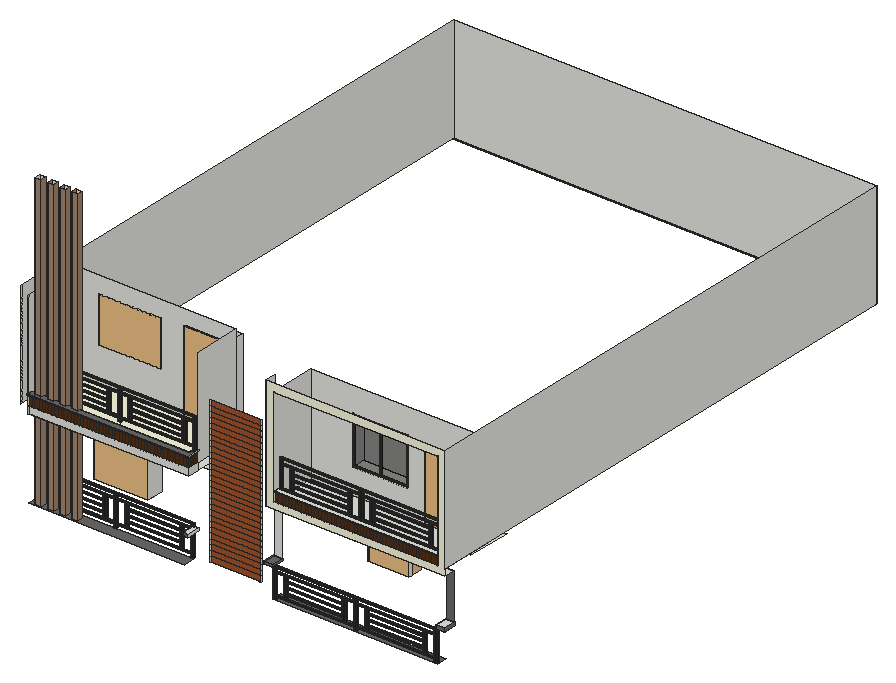
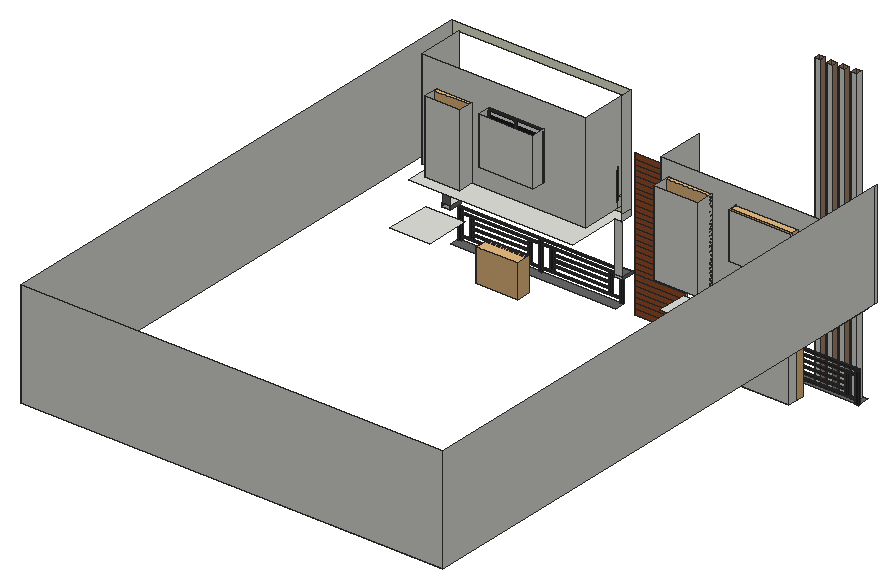
# SketchUp Ruby script. Lengths in inches.
U = 1.inch
M = Sketchup.active_model
def pt(a) = Geom::Point3d.new(a.map { |v| v * U })
def face(e, loops, mat)
  f = e.add_face(loops[0].map { |a| pt(a) })
  loops[1..].each { |l| e.add_face(l.map { |a| pt(a) }).erase! }
  f.material = f.back_material = mat if mat
  f
end
# faces: each face lists its corners as indices into pts; further lists are holes
def faces(e, pts, list, mat = nil) = list.each { |f| face(e, (f[0].is_a?(Array) ? f : [f]).map { |l| l.map { |i| pts[i] } }, mat) }
# xy, xz, yz: faces in a plane at the given z, y or x. An outline is a flat list of corners, or four numbers for a rectangle; further outlines are holes
def ring(l) = l.size == 4 ? [[l[0], l[1]], [l[2], l[1]], [l[2], l[3]], [l[0], l[3]]] : l.each_slice(2).to_a
def flat(e, list, mat, &to3) = list.each { |f| face(e, (f[0].is_a?(Array) ? f : [f]).map { |l| ring(l).map { |u, v| to3.(u, v) } }, mat) }
def xy(e, z, list, mat = nil) = flat(e, list, mat) { |x, y| [x, y, z] }
def xz(e, y, list, mat = nil) = flat(e, list, mat) { |x, z| [x, y, z] }
def yz(e, x, list, mat = nil) = flat(e, list, mat) { |y, z| [x, y, z] }
def lines(e, pts, list) = list.each { |a, b| e.add_line(pt(pts[a]), pt(pts[b])) }
# prism: a flat outline (further loops are holes) pulled along v
def prism(e, loops, v, mat = nil)
  f = face(e, loops, mat); d = Geom::Vector3d.new(v.map { |x| x * U })
  f.pushpull(f.normal.samedirection?(d) ? d.length : -d.length)
end
def box(e, o, s, mat = nil) = prism(e, [[o, [o[0] + s[0], o[1], o[2]], [o[0] + s[0], o[1] + s[1], o[2]], [o[0], o[1] + s[1], o[2]]]], [0, 0, s[2]], mat)
def at(x, y, z, deg = 0) = Geom::Transformation.translation(pt([x, y, z])) * Geom::Transformation.rotation(ORIGIN, Z_AXIS, deg.degrees)
def axes(o, x, y, z) = Geom::Transformation.new([*x, 0, *y, 0, *z, 0, *pt(o).to_a, 1])
def part(name) = M.definitions.add(name)
# library, detail: a bought-in or finely detailed component or shape, given as its bounding box
def library(name, o, s) = part(name).tap { |d| box(d.entities, o, s) }
def detail(e, o, s) = box(e.add_group.entities, o, s)
def put(e, d, t, mat = nil) = e.add_instance(d, t).tap { |i| i.material = mat if mat }
def group(e, t, mat = nil) = e.add_group.tap { |g| g.transformation = t; g.material = mat if mat }.entities
root = M.entities
M.materials.add("Glass_Tinted_Gray").color = [0, 0, 0]
M.materials["Glass_Tinted_Gray"].alpha = 0.125
M.materials.add("Painted Metal Railing").color = [35, 35, 35]
M.materials.add("Teddy_BraceletShadow ").color = [165, 134, 109]
M.materials.add("[0042_Sienna]").color = [160, 82, 45]
M.materials.add("[0049_Beige]").color = [245, 245, 220]
M.materials.add("[0134_DimGray]").color = [105, 105, 105]
M.materials.add("[0135_DarkGray]").color = [81, 81, 81]
M.materials.add("[Mirror 02]").color = [229, 229, 229]
M.materials.add("[Terrazzo Light Blue]").color = [196, 214, 227]
M.materials.add("[Wood Cherry Original]").color = [86, 49, 23]
c1 = part("Post")
box(c1.entities,[-0.75,-0.75,0],[1.5,1.5,34.5],"Painted Metal Railing")
c2 = part("Group43\#1")
box(c2.entities,[-0.75,0,0],[1.5,73.5,1.5],"Painted Metal Railing")
c3 = part("Group46\#2")
box(c3.entities,[-0.75,0.75,0],[1.5,34.5,1.5],"Painted Metal Railing")
c4 = part("Group49\#1")
box(c4.entities,[-0.75,0.75,0],[1.5,34.5,1.5],"Painted Metal Railing")
c5 = part("Group52\#1")
box(c5.entities,[-0.75,0.75,0],[1.5,34.5,1.5],"Painted Metal Railing")
c6 = part("Group55\#1")
box(c6.entities,[-0.75,0.75,0],[1.5,34.5,1.5],"Painted Metal Railing")
c7 = part("Inner Post")
box(c7.entities,[-0.75,-0.75,0],[1.5,1.5,23.5],"Painted Metal Railing")
c8 = part("Group59\#1")
box(c8.entities,[-0.75,0.75,0],[1.5,24.5,1.5],"Painted Metal Railing")
c9 = part("Group62\#1")
box(c9.entities,[-0.75,0.75,0],[1.5,24.5,1.5],"Painted Metal Railing")
c10 = part("Group65\#1")
box(c10.entities,[-0.75,0.75,0],[1.5,24.5,1.5],"Painted Metal Railing")
c11 = part("Inner Posts and Rails\#2")
put(c11.entities,c7,at(0,0,0,90))
put(c11.entities,c7,at(0,26,0,90))
put(c11.entities,c8,at(0,0,4.75))
put(c11.entities,c9,at(0,0,11))
put(c11.entities,c10,at(0,0,17.25))
c12 = part("Group69\#1")
box(c12.entities,[-0.75,0.75,0],[1.5,24.5,1.5],"Painted Metal Railing")
c13 = part("Group72\#1")
box(c13.entities,[-0.75,0.75,0],[1.5,24.5,1.5],"Painted Metal Railing")
c14 = part("Group75\#1")
box(c14.entities,[-0.75,0.75,0],[1.5,24.5,1.5],"Painted Metal Railing")
c15 = part("Inner Posts and Rails\#3")
put(c15.entities,c7,at(0,0,0,90))
put(c15.entities,c7,at(0,26,0,90))
put(c15.entities,c12,at(0,0,4.75))
put(c15.entities,c13,at(0,0,11))
put(c15.entities,c14,at(0,0,17.25))
c16 = part("Railing Assembly 14\#1")
put(c16.entities,c1,at(0,0,0))
put(c16.entities,c1,at(36,0,0))
put(c16.entities,c1,at(72,0,0))
put(c16.entities,c2,at(-0.75,0,34.5,-90))
put(c16.entities,c3,at(0,0,4,-90))
put(c16.entities,c4,at(36,0,4,-90))
put(c16.entities,c5,at(0,0,29,-90))
put(c16.entities,c6,at(36,0,29,-90))
put(c16.entities,c11,at(5,0,5.5,-90))
put(c16.entities,c15,at(41,0,5.5,-90))
c17 = library("Group\#6",[0,0,0],[8.07,62.0625,54])
c18 = library("PINTU 6 YA",[0,-0.6875,0],[35.83,8.07,80.71])
c19 = part("PENTEK_RP Fineline 50S_Sliding_DoorCase_E1")
box(c19.entities,[0,0,0],[1.51,3.66,99.27],"[0135_DarkGray]")
c20 = part("PENTEK_RP Fineline 50S_SlidingDooe_Case_E2")
box(c20.entities,[0,0,0],[96.25,3.66,1.51],"[0135_DarkGray]")
c21 = part("pentek_RP Fineline 50S_SlidingDoor_Case")
put(c21.entities,c19,at(97.76,0,0))
put(c21.entities,c20,at(1.51,0,0))
put(c21.entities,c19,at(0,0,0))
put(c21.entities,c20,at(1.51,0,97.76))
c22 = part("PENTEK_RP Fineline 50S_SlidingDoor_GlazingBead_2")
box(c22.entities,[0,0,0],[0.56,0.59,94.39],"[0135_DarkGray]")
c23 = part("PENTEK_RP Fineline 50S_SlidingDoor_Glass")
box(c23.entities,[0,0,0],[46.58,0.16,94.39],"Glass_Tinted_Gray")
c24 = part("PENTEK_RP Fineline 50S_SlidingDoor_GlazingBead")
box(c24.entities,[0,0,0],[45.47,0.59,0.56],"[0135_DarkGray]")
c25 = part("PENTEK_RP Fineline 50S_SlidingDoor_Leaf_E1")
xy(c25.entities,0,[[0,0,0.93,1.97],[0.93,1.57,1.49,1.97]],"[0135_DarkGray]")
xy(c25.entities,96.25,[[0,0,0.93,0,0.93,1.57,1.49,1.57,1.49,1.97,0,1.97]],"[0135_DarkGray]")
xz(c25.entities,0,[[0,0,0.93,96.25]],"[0135_DarkGray]")
xz(c25.entities,1.57,[[0.93,0,1.49,95.32],[0.93,95.32,1.49,96.25]],"[0135_DarkGray]")
xz(c25.entities,1.97,[[0,0,1.49,96.25]],"[0135_DarkGray]")
yz(c25.entities,0,[[0,0,1.97,96.25]],"[0135_DarkGray]")
yz(c25.entities,0.93,[[0,0,1.57,0.93],[0,0.93,1.57,95.32],[0,95.32,1.57,96.25]],"[0135_DarkGray]")
yz(c25.entities,1.49,[[1.57,0,1.97,95.32],[1.57,95.32,1.97,96.25]],"[0135_DarkGray]")
c26 = part("PENTEK_RP Fineline 50S_SlidingDoor_Leaf_E2")
xy(c26.entities,0,[[0,0,0,1.57,0.56,1.57,0.56,1.97,46.02,1.97,46.02,1.57,46.58,1.57,46.58,0]],"[0135_DarkGray]")
xy(c26.entities,0.93,[[0,0,46.58,1.57]],"[0135_DarkGray]")
xy(c26.entities,1.49,[[0.56,1.57,46.02,1.97]],"[0135_DarkGray]")
xz(c26.entities,0,[[0,0,46.58,0.93]],"[0135_DarkGray]")
xz(c26.entities,1.57,[[0,0,0.56,0.93],[46.02,0,46.58,0.93],[0.56,0.93,46.02,1.49]],"[0135_DarkGray]")
xz(c26.entities,1.97,[[0.56,0,46.02,1.49]],"[0135_DarkGray]")
yz(c26.entities,0,[[0,0,1.57,0.93]],"[0135_DarkGray]")
yz(c26.entities,0.56,[[1.57,0,1.97,0.93],[1.57,0.93,1.97,1.49]],"[0135_DarkGray]")
yz(c26.entities,46.02,[[1.57,0,1.97,0.93],[1.57,0.93,1.97,1.49]],"[0135_DarkGray]")
yz(c26.entities,46.58,[[0,0,1.57,0.93]],"[0135_DarkGray]")
c27 = part("PENTEK_RP Fineline S_SlidingDoor_Leaf1")
put(c27.entities,c22,at(0.93,0,0.93))
put(c27.entities,c22,at(46.96,0,0.93))
put(c27.entities,c23,at(1.49,1.42,0.93))
put(c27.entities,c24,at(1.49,0,0.93))
put(c27.entities,c23,at(1.49,0.59,0.93),"[Terrazzo Light Blue]")
put(c27.entities,c25,at(0,0,0))
put(c27.entities,c25,axes([48.44,0,0],[-1,0,0],[0,1,0],[0,0,1]))
put(c27.entities,c26,axes([0.93,0,96.25],[1,0,0],[0,1,0],[0,0,-1]))
put(c27.entities,c26,at(0.93,0,0))
put(c27.entities,c24,at(1.49,0,94.77))
c28 = part("PENTEK_RP Fineline 50S_SlidingDoor_Leaf2")
put(c28.entities,c23,at(1.49,1.42,0.93))
put(c28.entities,c24,at(1.49,0,94.77))
put(c28.entities,c22,at(46.96,0,0.93))
put(c28.entities,c23,at(1.49,0.59,0.93),"[Mirror 02]")
put(c28.entities,c22,at(0.93,0,0.93))
put(c28.entities,c25,at(0,0,0))
put(c28.entities,c25,axes([48.44,0,0],[-1,0,0],[0,1,0],[0,0,1]))
put(c28.entities,c24,at(1.49,0,0.93))
put(c28.entities,c26,axes([0.93,0,96.25],[1,0,0],[0,1,0],[0,0,-1]))
put(c28.entities,c26,at(0.93,0,0))
c29 = part("PENTEK - Slimmest Steel Sliding Door / Window\#1")
put(c29.entities,c21,at(0,-1.88,-0.09))
put(c29.entities,c27,at(1.51,-2.27,1.42))
put(c29.entities,c28,at(49.32,-0.3,1.42))
xy(root,140.3125,[[284.8125,3.0625,472,14.97]],"[0134_DimGray]")
xy(root,140.5625,[[[8,2.5625,185,15.9375],[13.71,5.07,20.52,11.88],[27.41,5.07,34.23,11.88],[41.12,5.07,47.93,11.88],[54.83,5.07,61.64,11.88]]],"[0134_DimGray]")
xy(root,143.51,[[203.35,17.0625,260.98,17.375]])
xy(root,154.08,[[41.11,54.5,102.36,73.625]])
xy(root,165.23,[[336.13,75.125,382.38,78.375]])
xy(root,170.625,[[184,1,185,15.9375],[185,1,189.625,3.0625],[189.625,1,190.625,3.0625],[185,3.0625,189.625,15.9375],[189.625,3.0625,190.625,15.9375]])
xy(root,173.625,[[184,1,190.625,15.9375],[275.8125,2.0625,276.8125,3.0625],[276.8125,2.0625,284.8125,15.9375],[284.8125,2.0625,285.8125,3.0625],[275.8125,3.0625,276.8125,15.9375],
  [284.8125,3.0625,285.8125,15.9375]])
xy(root,175.875,[[471,2.0625,472,3.0625],[472,2.0625,480,15.9375],[480,2.0625,481,3.0625],[471,3.0625,472,15.9375],[480,3.0625,481,15.9375]])
xy(root,175.875,[[275.8125,2.0625,285.8125,15.9375]],"[0134_DimGray]")
xy(root,179.9375,[[471,2.0625,481,15.9375]])
xy(root,202.54,[[336.13,75.125,382.38,78.375]])
xy(root,209.33,[[41.11,54.5,102.36,73.625]])
xy(root,209.5,[[134.5,54.5,175.6875,88.25]])
xy(root,211.875,[[407.59,75.125,452.27,125.625]])
xy(root,231.875,[[8,3.0625,189.625,54.5],[276.8125,3.0625,276.8125,15.9375,284.8125,15.9375,284.8125,75.125,472,75.125,472,15.9375,480,15.9375,480,3.0625]])
xy(root,239.875,[[8,3.0625,8,7.98,186.18,7.98,186.1875,15.9375,189.625,15.9375,189.625,3.0625],[286.5625,3.0625,472.04,4.25],[286.5625,4.25,472.04,9.0625],[286.5625,9.0625,472.04,9.0625,472.04,55.8125,455.32,55.8125,455.32,73,415.76,73,415.76,55.8125,286.5625,55.8125],[0,614.8125,480,615.9375]])
xy(root,239.875,[[8,7.98,186.18,7.98,186.1875,15.9375,189.625,15.9375,189.625,70.1875,180.3125,70.1875,180.3125,90.9375,131.125,90.9375,131.125,70.1875,8,70.1875]],"[0049_Beige]")
xy(root,249.875,[[286.5625,2.0625,472.04,4.25],[286.5625,4.25,472.04,9.0625]])
xy(root,250.875,[[286.5625,2.0625,472.04,9.0625]])
xy(root,251.875,[[8,0,190.625,3.0625],[8,3.0625,8,7.98,186.18,7.98,186.1875,15.9375,189.625,15.9375,189.625,3.0625],[189.625,3.0625,190.625,15.9375]])
xy(root,252.875,[[8,0,190.625,0,190.625,15.9375,186.1875,15.9375,186.18,7.98,8,7.98]],"[0134_DimGray]")
xy(root,269.32,[[334.19,55.8125,396.26,70.4375]])
xy(root,280.88,[[33.6,70.1875,103.97,80.1875]])
xz(root,0,[[8,251.875,190.625,252.875]],"[0134_DimGray]")
xz(root,1,[[184,170.625,190.625,173.625]],"[0134_DimGray]")
xz(root,2.0625,[[286.5625,249.875,472.04,250.875]])
xz(root,2.0625,[[275.8125,173.625,285.8125,175.875],[471,175.875,481,179.9375]],"[0134_DimGray]")
xz(root,3.0625,[[8,231.875,189.625,239.875]])
xz(root,3.0625,[[[276.8125,231.875,480,360],[286.5625,239.875,472.04,352]]],"[0049_Beige]")
xz(root,3.0625,[[8,239.875,11.63,251.875],[11.63,239.875,15.27,251.875],[15.27,239.875,18.9,251.875],[18.9,239.875,22.53,251.875],[22.53,239.875,26.16,251.875],
  [26.16,239.875,29.8,251.875],[29.8,239.875,33.43,251.875],[33.43,239.875,37.06,251.875],[37.06,239.875,40.69,251.875],[40.69,239.875,44.33,251.875],
  [44.33,239.875,47.96,251.875],[47.96,239.875,51.59,251.875],[51.59,239.875,55.22,251.875],[55.22,239.875,58.86,251.875],[58.86,239.875,62.49,251.875],
  [62.49,239.875,66.12,251.875],[66.12,239.875,69.75,251.875],[69.75,239.875,73.38,251.875],[73.38,239.875,77.02,251.875],[77.02,239.875,80.65,251.875],
  [80.65,239.875,84.28,251.875],[84.28,239.875,87.91,251.875],[87.91,239.875,91.55,251.875],[91.55,239.875,95.18,251.875],[95.18,239.875,98.8125,251.875],
  [98.8125,239.875,102.44,251.875],[102.44,239.875,106.08,251.875],[106.08,239.875,109.71,251.875],[109.71,239.875,113.34,251.875],[113.34,239.875,116.97,251.875],
  [116.97,239.875,120.61,251.875],[120.61,239.875,124.24,251.875],[124.24,239.875,127.87,251.875],[127.87,239.875,131.5,251.875],[131.5,239.875,135.14,251.875],
  [135.14,239.875,138.77,251.875],[138.77,239.875,142.4,251.875],[142.4,239.875,146.03,251.875],[146.03,239.875,149.67,251.875],[149.67,239.875,153.3,251.875],
  [153.3,239.875,156.93,251.875],[156.93,239.875,160.56,251.875],[160.56,239.875,164.2,251.875],[164.2,239.875,167.83,251.875],[167.83,239.875,171.46,251.875],
  [171.46,239.875,175.09,251.875],[175.09,239.875,178.73,251.875],[178.73,239.875,182.36,251.875],[182.36,239.875,185.99,251.875],[185.99,239.875,189.625,251.875]],"[Wood Cherry Original]")
xz(root,4.25,[[286.5625,239.875,290.27,249.875],[290.27,239.875,293.98,249.875],[293.98,239.875,297.69,249.875],[297.69,239.875,301.4,249.875],[301.4,239.875,305.11,249.875],
  [305.11,239.875,308.82,249.875],[308.82,239.875,312.53,249.875],[312.53,239.875,316.24,249.875],[316.24,239.875,319.95,249.875],[319.95,239.875,323.66,249.875],
  [323.66,239.875,327.37,249.875],[327.37,239.875,331.08,249.875],[331.08,239.875,334.79,249.875],[334.79,239.875,338.5,249.875],[338.5,239.875,342.21,249.875],
  [342.21,239.875,345.92,249.875],[345.92,239.875,349.63,249.875],[349.63,239.875,353.34,249.875],[353.34,239.875,357.05,249.875],[357.05,239.875,360.76,249.875],
  [360.76,239.875,364.47,249.875],[364.47,239.875,368.17,249.875],[368.17,239.875,371.88,249.875],[371.88,239.875,375.59,249.875],[375.59,239.875,379.3,249.875],
  [379.3,239.875,383.01,249.875],[383.01,239.875,386.72,249.875],[386.72,239.875,390.43,249.875],[390.43,239.875,394.14,249.875],[394.14,239.875,397.85,249.875],
  [397.85,239.875,401.5625,249.875],[401.5625,239.875,405.27,249.875],[405.27,239.875,408.98,249.875],[408.98,239.875,412.69,249.875],[412.69,239.875,416.4,249.875],
  [416.4,239.875,420.11,249.875],[420.11,239.875,423.82,249.875],[423.82,239.875,427.53,249.875],[427.53,239.875,431.24,249.875],[431.24,239.875,434.95,249.875],
  [434.95,239.875,438.66,249.875],[438.66,239.875,442.37,249.875],[442.37,239.875,446.08,249.875],[446.08,239.875,449.79,249.875],[449.79,239.875,453.49,249.875],
  [453.49,239.875,457.2,249.875],[457.2,239.875,460.91,249.875],[460.91,239.875,464.625,249.875],[464.625,239.875,468.33,249.875],[468.33,239.875,472.04,249.875]],"[Wood Cherry Original]")
xz(root,5.07,[[13.71,140.5625,20.52,472.625],[27.41,140.5625,34.23,472.625],[41.12,140.5625,47.93,471.9375],[54.83,140.5625,61.64,472.625]],"Teddy_BraceletShadow ")
xz(root,7.98,[[8,239.875,186.18,251.875],[8,251.875,186.18,252.875]])
xz(root,9.0625,[[286.5625,239.875,472.04,249.875],[286.5625,249.875,472.04,250.875]])
xz(root,11.88,[[13.71,140.5625,20.52,472.625],[27.41,140.5625,34.23,472.625],[41.12,140.5625,47.93,471.9375],[54.83,140.5625,61.64,472.625]])
xz(root,15.9375,[[184,170.625,189.625,173.625],[189.625,170.625,190.625,173.625],[275.8125,173.625,284.8125,175.875],[284.8125,173.625,285.8125,175.875],[276.8125,175.875,284.8125,231.875],
  [471,175.875,472,179.9375],[472,175.875,480,179.9375],[480,175.875,481,179.9375],[186.1875,239.875,189.625,251.875],[186.1875,251.875,189.625,252.875],
  [189.625,251.875,190.625,252.875]])
xz(root,15.9375,[[472,179.9375,480,231.875]],"[0134_DimGray]")
xz(root,17.0625,[[203.35,143.51,260.98,149.39],[203.35,149.39,260.98,155.26],[203.35,155.26,260.98,161.14],[203.35,161.14,260.98,167.02],[203.35,167.02,260.98,172.89],
  [203.35,172.89,260.98,178.77],[203.35,178.77,260.98,184.65],[203.35,184.65,260.98,190.52],[203.35,190.52,260.98,196.4],[203.35,196.4,260.98,202.28],
  [203.35,202.28,260.98,208.16],[203.35,208.16,260.98,214.03],[203.35,214.03,260.98,219.91],[203.35,219.91,260.98,225.79],[203.35,225.79,260.98,231.66],
  [203.35,231.66,260.98,237.54],[203.35,237.54,260.98,243.42],[203.35,243.42,260.98,249.3],[203.35,249.3,260.98,255.17],[203.35,255.17,260.98,261.05],
  [203.35,261.05,260.98,266.93],[203.35,266.93,260.98,272.8],[203.35,272.8,260.98,278.68],[203.35,278.68,260.98,284.56],[203.35,284.56,260.98,290.44],
  [203.35,290.44,260.98,296.3125],[203.35,296.3125,260.98,302.19],[203.35,302.19,260.98,308.07]],"[0042_Sienna]")
xz(root,55.8125,[[[286.5625,239.875,415.76,239.875,415.76,321.9375,455.32,321.9375,455.32,239.875,472.04,239.875,472.04,352,286.5625,352],[334.19,269.32,396.26,323.32]]])
xz(root,70.1875,[[[8,239.875,131.125,239.875,131.125,335.1875,180.3125,335.1875,180.3125,239.875,189.625,239.875,189.625,352,8,352],[33.6,280.88,103.97,332.51]]])
xz(root,70.4375,[[334.19,269.32,396.26,323.32]])
xz(root,73,[[415.76,239.875,455.32,321.9375]])
xz(root,73.625,[[41.11,154.08,102.36,209.33]])
xz(root,78.375,[[336.13,165.23,382.38,202.54]])
xz(root,80.1875,[[33.6,280.88,103.97,332.51]])
xz(root,90.9375,[[131.125,239.875,180.3125,335.1875]])
xz(root,615.9375,[[0,239.875,480,360]])
yz(root,0,[[1,239.875,3.0625,360],[3.0625,239.875,615.9375,360]])
yz(root,8,[[1,231.875,3.0625,239.875],[1,239.875,3.0625,251.875],[3.0625,239.875,7.98,251.875],[7.98,239.875,70.1875,239.875,70.1875,352,3.0625,352,3.0625,252.875,7.98,252.875],[0,251.875,1,252.875],
  [1,251.875,7.98,252.875],[1,252.875,3.0625,352]])
yz(root,13.71,[[5.07,140.5625,11.88,472.625]])
yz(root,20.52,[[5.07,140.5625,11.88,472.625]],"Teddy_BraceletShadow ")
yz(root,27.41,[[5.07,140.5625,11.88,472.625]],"Teddy_BraceletShadow ")
yz(root,33.6,[[70.1875,280.88,80.1875,332.51]])
yz(root,34.23,[[5.07,140.5625,11.88,472.625]],"Teddy_BraceletShadow ")
yz(root,41.11,[[54.5,154.08,73.625,209.33]])
yz(root,41.12,[[5.07,140.5625,11.88,471.9375]],"Teddy_BraceletShadow ")
yz(root,47.93,[[5.07,140.5625,11.88,471.9375]],"Teddy_BraceletShadow ")
yz(root,54.83,[[5.07,140.5625,11.88,472.625]],"Teddy_BraceletShadow ")
yz(root,61.64,[[5.07,140.5625,11.88,472.625]],"Teddy_BraceletShadow ")
yz(root,102.36,[[54.5,154.08,73.625,209.33]])
yz(root,103.97,[[70.1875,280.88,80.1875,332.51]])
yz(root,131.125,[[70.1875,239.875,90.9375,335.1875]])
yz(root,180.3125,[[70.1875,239.875,90.9375,335.1875]])
yz(root,184,[[1,170.625,15.9375,173.625]],"[0134_DimGray]")
yz(root,189.625,[[3.0625,231.875,15.9375,239.875],[15.9375,239.875,70.1875,352]])
yz(root,189.625,[[3.0625,239.875,5.21,251.875],[5.21,239.875,7.35,251.875],[7.35,239.875,9.5,251.875],[9.5,239.875,11.65,251.875],[11.65,239.875,13.79,251.875],
  [13.79,239.875,15.9375,251.875]],"[Wood Cherry Original]")
yz(root,190.625,[[1,170.625,15.9375,173.625],[0,251.875,15.9375,252.875]])
yz(root,203.35,[[15.9375,143.51,17.0625,149.39],[15.9375,149.39,17.0625,155.26],[15.9375,155.26,17.0625,161.14],[15.9375,161.14,17.0625,167.02],[15.9375,167.02,17.0625,172.89],
  [15.9375,172.89,17.0625,178.77],[15.9375,178.77,17.0625,184.65],[15.9375,184.65,17.0625,190.52],[15.9375,190.52,17.0625,196.4],[15.9375,196.4,17.0625,202.28],
  [15.9375,202.28,17.0625,208.16],[15.9375,208.16,17.0625,214.03],[15.9375,214.03,17.0625,219.91],[15.9375,219.91,17.0625,225.79],[15.9375,225.79,17.0625,231.66],
  [15.9375,231.66,17.0625,237.54],[15.9375,237.54,17.0625,243.42],[15.9375,243.42,17.0625,249.3],[15.9375,249.3,17.0625,255.17],[15.9375,255.17,17.0625,261.05],
  [15.9375,261.05,17.0625,266.93],[15.9375,266.93,17.0625,272.8],[15.9375,272.8,17.0625,278.68],[15.9375,278.68,17.0625,284.56],[15.9375,284.56,17.0625,290.44],
  [15.9375,290.44,17.0625,296.3125],[15.9375,296.3125,17.0625,302.19],[15.9375,302.19,17.0625,308.07]])
yz(root,260.98,[[15.9375,143.51,17.0625,149.39],[15.9375,149.39,17.0625,155.26],[15.9375,155.26,17.0625,161.14],[15.9375,161.14,17.0625,167.02],[15.9375,167.02,17.0625,172.89],
  [15.9375,172.89,17.0625,178.77],[15.9375,178.77,17.0625,184.65],[15.9375,184.65,17.0625,190.52],[15.9375,190.52,17.0625,196.4],[15.9375,196.4,17.0625,202.28],
  [15.9375,202.28,17.0625,208.16],[15.9375,208.16,17.0625,214.03],[15.9375,214.03,17.0625,219.91],[15.9375,219.91,17.0625,225.79],[15.9375,225.79,17.0625,231.66],
  [15.9375,231.66,17.0625,237.54],[15.9375,237.54,17.0625,243.42],[15.9375,243.42,17.0625,249.3],[15.9375,249.3,17.0625,255.17],[15.9375,255.17,17.0625,261.05],
  [15.9375,261.05,17.0625,266.93],[15.9375,266.93,17.0625,272.8],[15.9375,272.8,17.0625,278.68],[15.9375,278.68,17.0625,284.56],[15.9375,284.56,17.0625,290.44],
  [15.9375,290.44,17.0625,296.3125],[15.9375,296.3125,17.0625,302.19],[15.9375,302.19,17.0625,308.07]])
yz(root,275.8125,[[2.0625,173.625,15.9375,175.875]],"[0134_DimGray]")
yz(root,276.8125,[[3.0625,231.875,15.9375,239.875],[3.0625,239.875,15.9375,360]])
yz(root,285.8125,[[2.0625,173.625,15.9375,175.875]],"[0134_DimGray]")
yz(root,286.5625,[[3.0625,239.875,4.25,249.875],[9.0625,239.875,55.8125,239.875,55.8125,352,3.0625,352,3.0625,250.875,9.0625,250.875],[4.25,239.875,9.0625,249.875],[2.0625,249.875,3.0625,250.875],[3.0625,249.875,9.0625,250.875]])
yz(root,334.19,[[55.8125,269.32,70.4375,323.32]])
yz(root,336.13,[[75.125,165.23,78.375,202.54]])
yz(root,382.38,[[75.125,165.23,78.375,202.54]])
yz(root,396.26,[[55.8125,269.32,70.4375,323.32]])
yz(root,415.76,[[55.8125,239.875,73,321.9375]])
yz(root,455.32,[[55.8125,239.875,73,321.9375]])
yz(root,471,[[2.0625,175.875,15.9375,179.9375]],"[0134_DimGray]")
yz(root,472.04,[[3.0625,239.875,4.25,249.875],[9.0625,239.875,9.0625,250.875,3.0625,250.875,3.0625,352,55.8125,352,55.8125,239.875],[4.25,239.875,9.0625,249.875],[2.0625,249.875,3.0625,250.875],[3.0625,249.875,9.0625,250.875]])
yz(root,480,[[3.0625,239.875,615.9375,360]])
yz(root,481,[[2.0625,175.875,15.9375,179.9375]],"[0134_DimGray]")
p = [[186.1875,15.9375,239.875],[186.18,7.98,239.875],[186.18,7.98,251.875],[186.1875,15.9375,251.875],[186.18,7.98,252.875],[186.1875,15.9375,252.875],
  [4.56,7.98,239.875],[8,7.98,239.875]]
faces(root,p,[[0,1,2,3],[3,2,4,5]])
lines(root,p,[[6,7]])
put(root,c16,axes([286.72,3.8125,140.3125],[2.54677,0,0],[0,1,0],[0,0,0.96]))
put(root,c16,axes([8.94,16.6875,140.5625],[2.42,0,0],[0,1,0],[0,0,1]))
put(root,c17,axes([102.36,54.5,154.08],[0,1,0],[-0.98691,0,0],[0,0,1.02315]))
put(root,c17,axes([382.38,75.125,165.23],[0,1.9706,0],[-0.7644,0,0],[0,0,0.69097]))
put(root,c18,axes([131.125,70.1875,239.875],[1.37281,0,0],[0,0.5,0],[0,0,1.18095]))
put(root,c18,axes([415.76,55.8125,239.875],[1.10418,0,0],[0,0.5,0],[0,0,1.01677]))
put(root,c16,axes([288.47,9.8125,246.875],[2.54392,0,0],[0,1,0],[0,0,1]))
put(root,c16,axes([17.95,12.42,252.875],[2.3735,0,0],[0,1,0],[0,0,1]))
put(root,c29,axes([334.19,56.41,269.37],[0.62517,0,0],[0,0.26184,0],[0,0,0.54396]))
put(root,c17,axes([103.97,70.1875,280.88],[0,1,0],[-1.13394,0,0],[0,0,0.97]))
